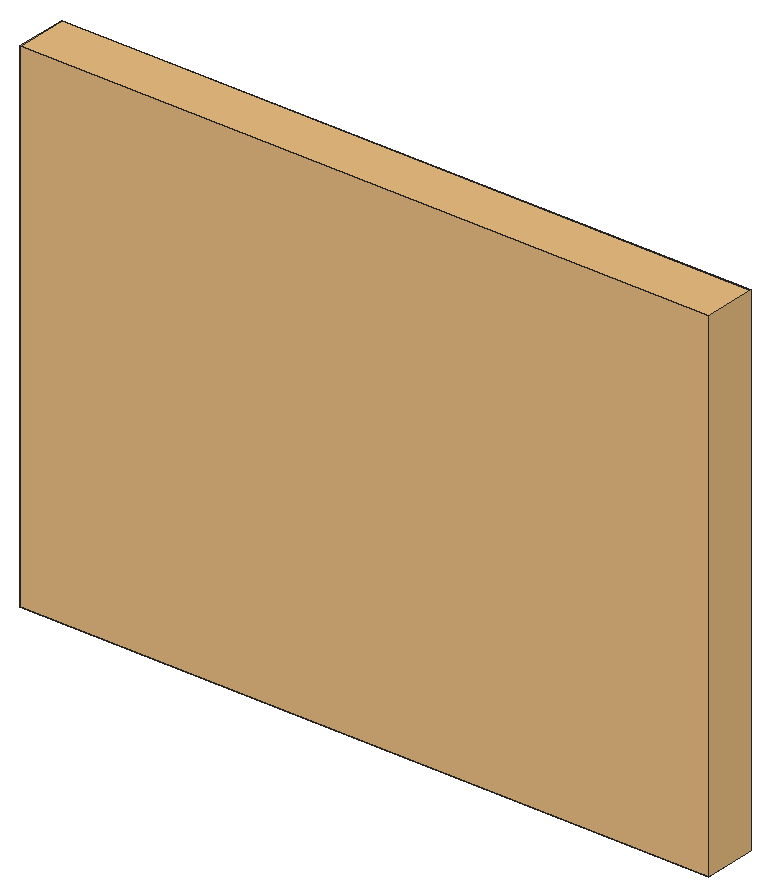
# SketchUp Ruby script. Lengths in inches.
U = 1.inch
M = Sketchup.active_model
def pt(a) = Geom::Point3d.new(a.map { |v| v * U })
def face(e, loops, mat)
  f = e.add_face(loops[0].map { |a| pt(a) })
  loops[1..].each { |l| e.add_face(l.map { |a| pt(a) }).erase! }
  f.material = f.back_material = mat if mat
  f
end
# faces: each face lists its corners as indices into pts; further lists are holes
def faces(e, pts, list, mat = nil) = list.each { |f| face(e, (f[0].is_a?(Array) ? f : [f]).map { |l| l.map { |i| pts[i] } }, mat) }
# xy, xz, yz: faces in a plane at the given z, y or x. An outline is a flat list of corners, or four numbers for a rectangle; further outlines are holes
def ring(l) = l.size == 4 ? [[l[0], l[1]], [l[2], l[1]], [l[2], l[3]], [l[0], l[3]]] : l.each_slice(2).to_a
def flat(e, list, mat, &to3) = list.each { |f| face(e, (f[0].is_a?(Array) ? f : [f]).map { |l| ring(l).map { |u, v| to3.(u, v) } }, mat) }
def xy(e, z, list, mat = nil) = flat(e, list, mat) { |x, y| [x, y, z] }
def xz(e, y, list, mat = nil) = flat(e, list, mat) { |x, z| [x, y, z] }
def yz(e, x, list, mat = nil) = flat(e, list, mat) { |y, z| [x, y, z] }
def lines(e, pts, list) = list.each { |a, b| e.add_line(pt(pts[a]), pt(pts[b])) }
# prism: a flat outline (further loops are holes) pulled along v
def prism(e, loops, v, mat = nil)
  f = face(e, loops, mat); d = Geom::Vector3d.new(v.map { |x| x * U })
  f.pushpull(f.normal.samedirection?(d) ? d.length : -d.length)
end
def box(e, o, s, mat = nil) = prism(e, [[o, [o[0] + s[0], o[1], o[2]], [o[0] + s[0], o[1] + s[1], o[2]], [o[0], o[1] + s[1], o[2]]]], [0, 0, s[2]], mat)
def at(x, y, z, deg = 0) = Geom::Transformation.translation(pt([x, y, z])) * Geom::Transformation.rotation(ORIGIN, Z_AXIS, deg.degrees)
def axes(o, x, y, z) = Geom::Transformation.new([*x, 0, *y, 0, *z, 0, *pt(o).to_a, 1])
def part(name) = M.definitions.add(name)
# library, detail: a bought-in or finely detailed component or shape, given as its bounding box
def library(name, o, s) = part(name).tap { |d| box(d.entities, o, s) }
def detail(e, o, s) = box(e.add_group.entities, o, s)
def put(e, d, t, mat = nil) = e.add_instance(d, t).tap { |i| i.material = mat if mat }
def group(e, t, mat = nil) = e.add_group.tap { |g| g.transformation = t; g.material = mat if mat }.entities
root = M.entities
# 65 loose lines left out
detail(root,[0,0,0],[140,10.75,102])
